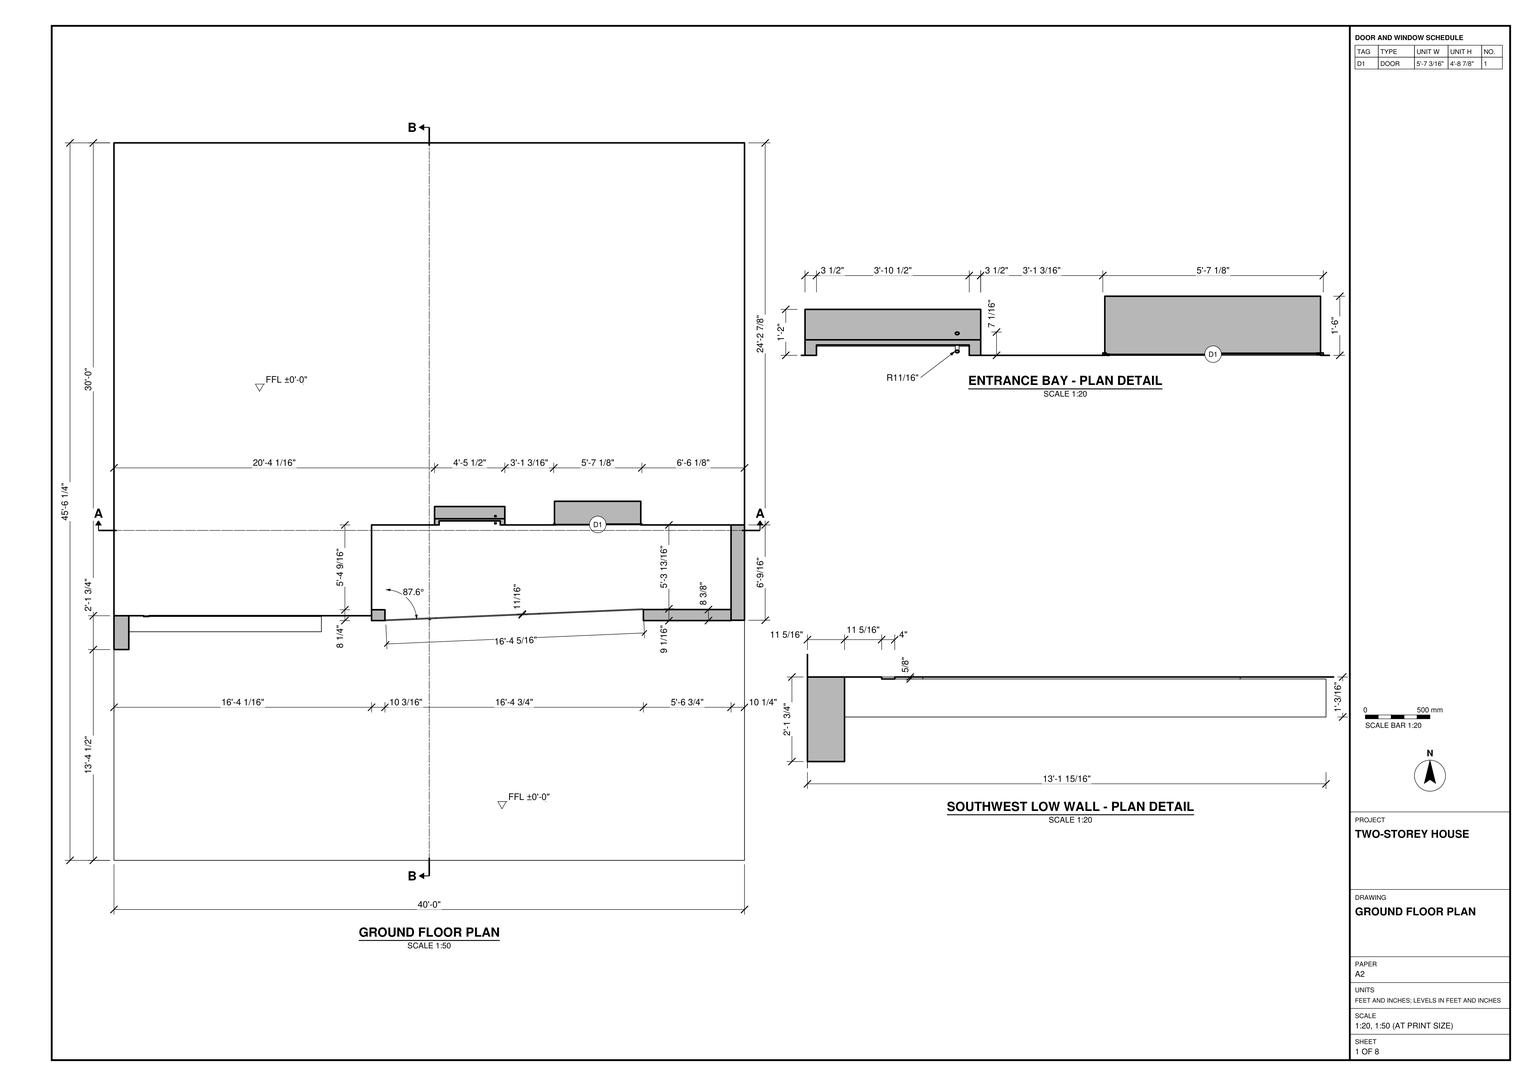
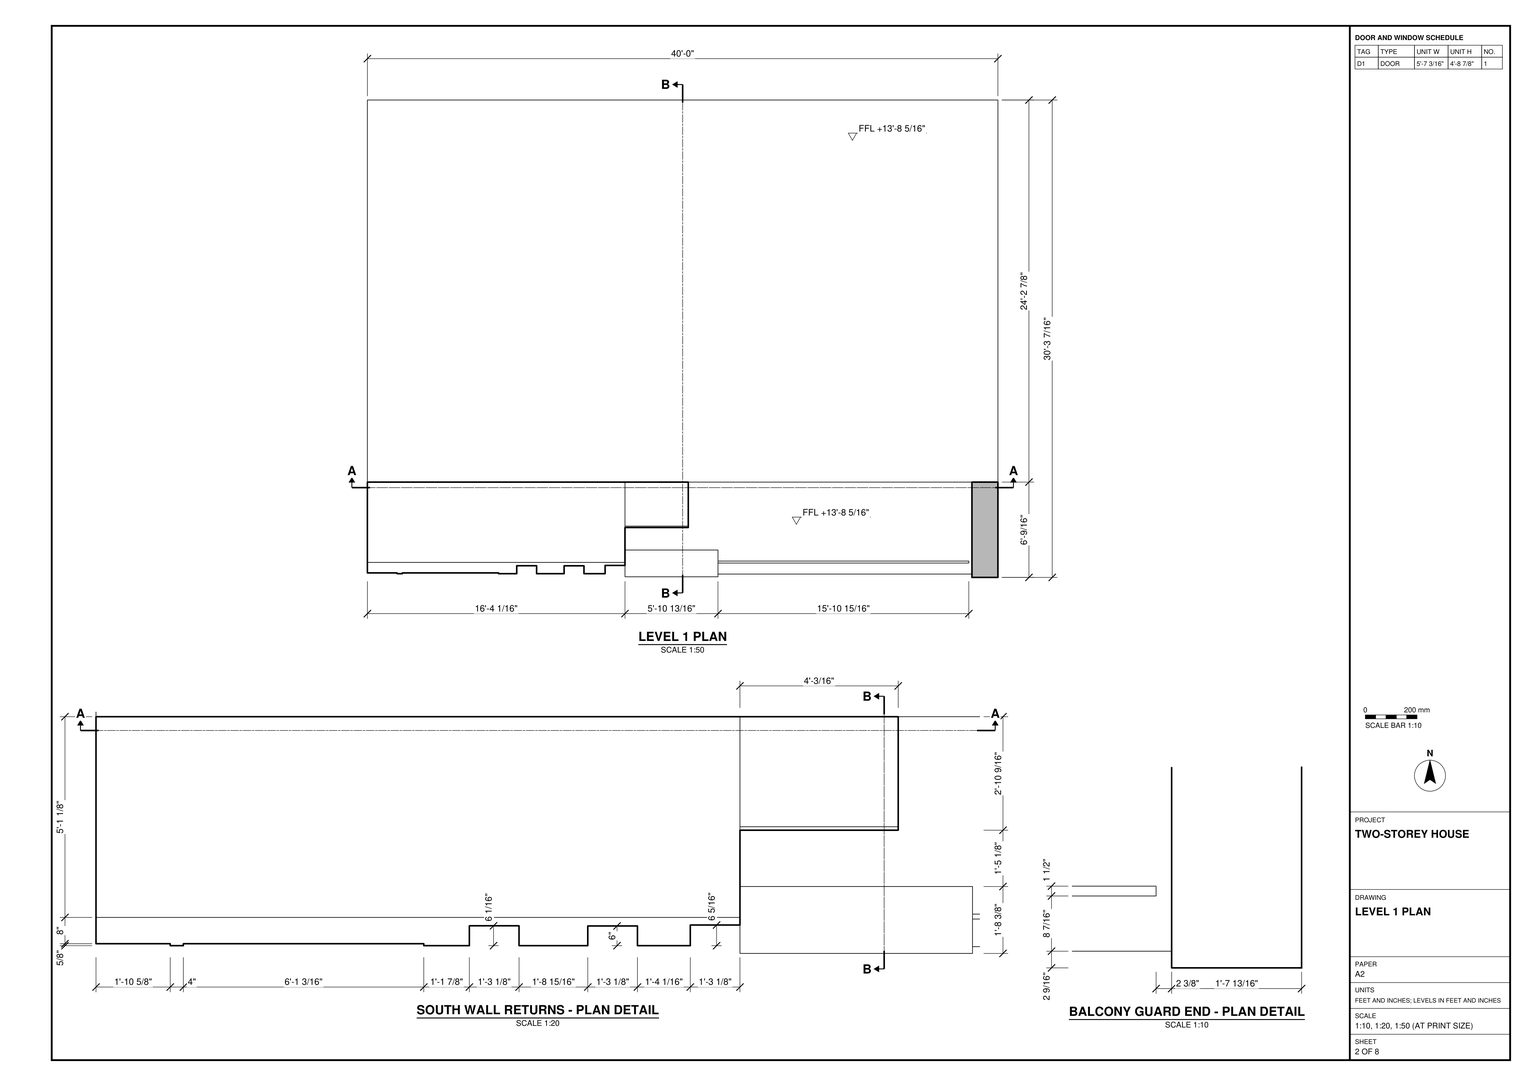
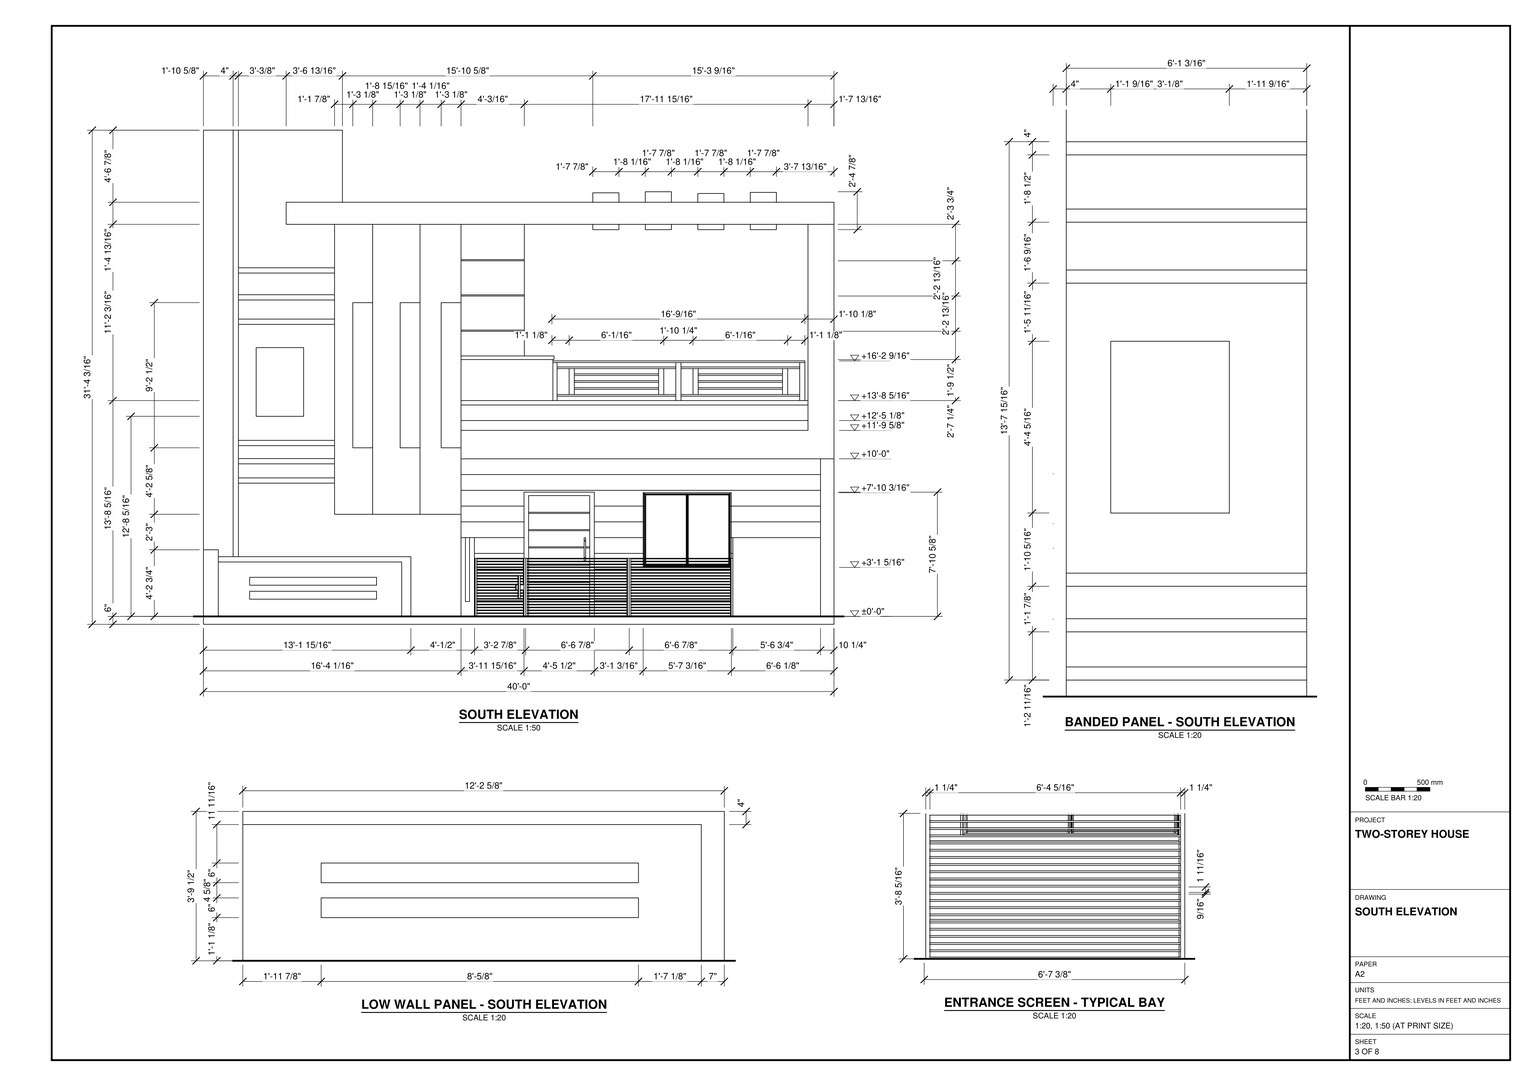
Model the two-storey house in SketchUp using task_files/diagram_01.pdf. Work in feet and inches. The overall model is 40'-0" wide, 45'-6 1/4" deep and 31'-4 3/16" high, including the base slab. Set the ground floor at ±0'-0" and the upper floor at +13'-8 5/16".

Use the plans to distinguish the full base slab from the smaller house footprint. Match the wall thicknesses, returns, floor slabs and roof outline to the drawings. On the south side, set the entrance back from the screen and follow the slight angle of the screen in plan. Include the framed sliding door, the horizontal slats and the separate low wall at the southwest corner with its two long inset strips.

Use the south elevation together with the upper-floor plan to shape the tall banded panel, the projecting vertical wall returns and the open balcony bay. Model the balcony slab and guard, the end support and the long overhead member with its short crosspieces. Include stairs, built-in joinery and main furniture only where shown. Decor and loose items may be any suitable library components.

Keep shell elements such as walls, slabs and roof separate as groups or components, and do the same for each furniture or joinery piece. Use components for repeated parts. Save one SketchUp model as output_files/two_storey_house_with_its_screened_entrance_and_balcony.skp.

# SketchUp Ruby script. Lengths in inches.
U = 1.inch
M = Sketchup.active_model
def pt(a) = Geom::Point3d.new(a.map { |v| v * U })
def face(e, loops, mat)
  f = e.add_face(loops[0].map { |a| pt(a) })
  loops[1..].each { |l| e.add_face(l.map { |a| pt(a) }).erase! }
  f.material = f.back_material = mat if mat
  f
end
# faces: each face lists its corners as indices into pts; further lists are holes
def faces(e, pts, list, mat = nil) = list.each { |f| face(e, (f[0].is_a?(Array) ? f : [f]).map { |l| l.map { |i| pts[i] } }, mat) }
# xy, xz, yz: faces in a plane at the given z, y or x. An outline is a flat list of corners, or four numbers for a rectangle; further outlines are holes
def ring(l) = l.size == 4 ? [[l[0], l[1]], [l[2], l[1]], [l[2], l[3]], [l[0], l[3]]] : l.each_slice(2).to_a
def flat(e, list, mat, &to3) = list.each { |f| face(e, (f[0].is_a?(Array) ? f : [f]).map { |l| ring(l).map { |u, v| to3.(u, v) } }, mat) }
def xy(e, z, list, mat = nil) = flat(e, list, mat) { |x, y| [x, y, z] }
def xz(e, y, list, mat = nil) = flat(e, list, mat) { |x, z| [x, y, z] }
def yz(e, x, list, mat = nil) = flat(e, list, mat) { |y, z| [x, y, z] }
def lines(e, pts, list) = list.each { |a, b| e.add_line(pt(pts[a]), pt(pts[b])) }
# prism: a flat outline (further loops are holes) pulled along v
def prism(e, loops, v, mat = nil)
  f = face(e, loops, mat); d = Geom::Vector3d.new(v.map { |x| x * U })
  f.pushpull(f.normal.samedirection?(d) ? d.length : -d.length)
end
def box(e, o, s, mat = nil) = prism(e, [[o, [o[0] + s[0], o[1], o[2]], [o[0] + s[0], o[1] + s[1], o[2]], [o[0], o[1] + s[1], o[2]]]], [0, 0, s[2]], mat)
def at(x, y, z, deg = 0) = Geom::Transformation.translation(pt([x, y, z])) * Geom::Transformation.rotation(ORIGIN, Z_AXIS, deg.degrees)
def axes(o, x, y, z) = Geom::Transformation.new([*x, 0, *y, 0, *z, 0, *pt(o).to_a, 1])
def part(name) = M.definitions.add(name)
# library, detail: a bought-in or finely detailed component or shape, given as its bounding box
def library(name, o, s) = part(name).tap { |d| box(d.entities, o, s) }
def detail(e, o, s) = box(e.add_group.entities, o, s)
def put(e, d, t, mat = nil) = e.add_instance(d, t).tap { |i| i.material = mat if mat }
def group(e, t, mat = nil) = e.add_group.tap { |g| g.transformation = t; g.material = mat if mat }.entities
root = M.entities
M.materials.add("Glass_Tinted_Gray").color = [0, 0, 0]
M.materials["Glass_Tinted_Gray"].alpha = 0.125
M.materials.add("Painted Metal Railing").color = [35, 35, 35]
M.materials.add("[0042_Sienna]").color = [160, 82, 45]
M.materials.add("[0129_WhiteSmoke]").color = [245, 245, 245]
M.materials.add("[0135_DarkGray]").color = [81, 81, 81]
M.materials.add("[Carrera Marble]").color = [207, 207, 207]
M.materials.add("[Color G01]").color = [204, 255, 204]
M.materials.add("[Color H01]").color = [204, 255, 255]
M.materials.add("[Color M00]").color = [255, 255, 255]
M.materials.add("[Color M04]").color = [142, 142, 142]
M.materials.add("[Color M05]").color = [114, 114, 114]
M.materials.add("[Color M06]").color = [86, 86, 86]
M.materials.add("[Color M07]").color = [58, 58, 58]
M.materials.add("[Metal_Corrogated_Shiny]2").color = [114, 114, 114]
M.materials.add("[Mirror 02]").color = [229, 229, 229]
M.materials.add("[Sandstone]").color = [118, 81, 52]
M.materials.add("[Terrazzo Light Blue]").color = [196, 214, 227]
M.materials.add("[Wood Veneer 01]").color = [119, 70, 35]
M.materials.add("[Wood Veneer 01]1").color = [120, 70, 37]
c1 = part("Post")
box(c1.entities,[-0.75,-0.75,0],[1.5,1.5,34.5],"Painted Metal Railing")
c2 = part("Group43\#1")
box(c2.entities,[-0.75,0,0],[1.5,73.5,1.5],"Painted Metal Railing")
c3 = part("Group46\#1")
box(c3.entities,[-0.75,0.75,0],[1.5,34.5,1.5],"Painted Metal Railing")
c4 = part("Group49\#1")
box(c4.entities,[-0.75,0.75,0],[1.5,34.5,1.5],"Painted Metal Railing")
c5 = part("Group52\#1")
box(c5.entities,[-0.75,0.75,0],[1.5,34.5,1.5],"Painted Metal Railing")
c6 = part("Group55\#1")
box(c6.entities,[-0.75,0.75,0],[1.5,34.5,1.5],"Painted Metal Railing")
c7 = part("Inner Post")
box(c7.entities,[-0.75,-0.75,0],[1.5,1.5,23.5],"Painted Metal Railing")
c8 = part("Group59\#1")
box(c8.entities,[-0.75,0.75,0],[1.5,24.5,1.5],"Painted Metal Railing")
c9 = part("Group62\#1")
box(c9.entities,[-0.75,0.75,0],[1.5,24.5,1.5],"Painted Metal Railing")
c10 = part("Group65\#1")
box(c10.entities,[-0.75,0.75,0],[1.5,24.5,1.5],"Painted Metal Railing")
c11 = part("Inner Posts and Rails\#2")
put(c11.entities,c7,at(0,0,0,90))
put(c11.entities,c7,at(0,26,0,90))
put(c11.entities,c8,at(0,0,4.75))
put(c11.entities,c9,at(0,0,11))
put(c11.entities,c10,at(0,0,17.25))
c12 = part("Group69\#1")
box(c12.entities,[-0.75,0.75,0],[1.5,24.5,1.5],"Painted Metal Railing")
c13 = part("Group72\#1")
box(c13.entities,[-0.75,0.75,0],[1.5,24.5,1.5],"Painted Metal Railing")
c14 = part("Group75\#1")
box(c14.entities,[-0.75,0.75,0],[1.5,24.5,1.5],"Painted Metal Railing")
c15 = part("Inner Posts and Rails\#3")
put(c15.entities,c7,at(0,0,0,90))
put(c15.entities,c7,at(0,26,0,90))
put(c15.entities,c12,at(0,0,4.75))
put(c15.entities,c13,at(0,0,11))
put(c15.entities,c14,at(0,0,17.25))
c16 = part("Railing Assembly 14\#1")
put(c16.entities,c1,at(0,0,0))
put(c16.entities,c1,at(36,0,0))
put(c16.entities,c1,at(72,0,0))
put(c16.entities,c2,at(-0.75,0,34.5,-90))
put(c16.entities,c3,at(0,0,4,-90))
put(c16.entities,c4,at(36,0,4,-90))
put(c16.entities,c5,at(0,0,29,-90))
put(c16.entities,c6,at(36,0,29,-90))
put(c16.entities,c11,at(5,0,5.5,-90))
put(c16.entities,c15,at(41,0,5.5,-90))
c17 = part("Group\#1")
xy(c17.entities,0,[[0.39,1.57,0.29,1.59,0.2,1.63,0.12,1.69,0.05,1.77,0.01,1.87,0,1.97,0.01,2.07,0.05,2.17,0.12,2.25,0.2,2.31,0.29,2.35,0.39,2.36,0.5,2.35,0.59,2.31,0.67,2.25,0.73,2.17,0.77,2.07,0.79,1.97,0.77,1.87,0.73,1.77,0.67,1.69,0.59,1.63,0.5,1.59],[0.39,13.39,0.29,13.4,0.2,13.4375,0.12,13.5,0.05,13.58,0.01,13.68,0,13.78,0.01,13.88,0.05,13.98,0.12,14.06,0.2,14.12,0.29,14.16,0.39,14.17,0.5,14.16,0.59,14.12,0.67,14.06,0.73,13.98,0.77,13.88,0.79,13.78,0.77,13.68,0.73,13.58,0.67,13.5,0.59,13.4375,0.5,13.4]])
xy(c17.entities,1.97,[[0.39,1.57,0.39,2.36,0.29,2.35,0.2,2.31,0.12,2.25,0.05,2.17,0.01,2.07,0,1.97,0.01,1.87,0.05,1.77,0.12,1.69,0.2,1.63,0.29,1.59],[0.39,1.57,0.5,1.59,0.59,1.63,0.67,1.69,0.73,1.77,0.77,1.87,0.79,1.97,0.77,2.07,0.73,2.17,0.67,2.25,0.59,2.31,0.5,2.35,0.39,2.36],[0.39,13.39,0.39,14.17,0.29,14.16,0.2,14.12,0.12,14.06,0.05,13.98,0.01,13.88,0,13.78,0.01,13.68,0.05,13.58,0.12,13.5,0.2,13.4375,0.29,13.4],[0.39,13.39,0.5,13.4,0.59,13.4375,0.67,13.5,0.73,13.58,0.77,13.68,0.79,13.78,0.77,13.88,0.73,13.98,0.67,14.06,0.59,14.12,0.5,14.16,0.39,14.17]])
xz(c17.entities,0,[[0.39,1.57,0.5,1.59,0.59,1.63,0.67,1.69,0.73,1.77,0.77,1.87,0.79,1.97,0.77,2.07,0.73,2.17,0.67,2.25,0.59,2.31,0.5,2.35,0.39,2.36,0.29,2.35,0.2,2.31,0.12,2.25,0.05,2.17,0.01,2.07,0,1.97,0.01,1.87,0.05,1.77,0.12,1.69,0.2,1.63,0.29,1.59]])
xz(c17.entities,15.75,[[0.39,1.57,0.29,1.59,0.2,1.63,0.12,1.69,0.05,1.77,0.01,1.87,0,1.97,0.01,2.07,0.05,2.17,0.12,2.25,0.2,2.31,0.29,2.35,0.39,2.36,0.5,2.35,0.59,2.31,0.67,2.25,0.73,2.17,0.77,2.07,0.79,1.97,0.77,1.87,0.73,1.77,0.67,1.69,0.59,1.63,0.5,1.59]])
p = [[0.12,1.69,0],[0.2,1.63,0],[0.2,1.63,1.63],[0.2,1.63,1.97],[0.12,1.69,1.97],[0.12,1.69,1.69],
  [0.29,1.59,0],[0.29,1.59,1.59],[0.29,1.59,1.97],[0.39,1.57,0],[0.39,1.57,1.57],[0.39,1.57,1.97],
  [0.5,1.59,0],[0.5,1.59,1.59],[0.5,1.59,1.97],[0.59,1.63,0],[0.59,1.63,1.63],[0.59,1.63,1.97],
  [0.67,1.69,0],[0.67,1.69,1.69],[0.67,1.69,1.97],[0.05,1.77,0],[0.05,1.77,1.97],[0.05,1.77,1.77],
  [0.73,1.77,0],[0.73,1.77,1.77],[0.73,1.77,1.97],[0.01,1.87,0],[0.01,1.87,1.97],[0.01,1.87,1.87],
  [0.77,1.87,0],[0.77,1.87,1.87],[0.77,1.87,1.97],[0,1.97,0],[0,1.97,1.97],[0.79,1.97,0],
  [0.79,1.97,1.97],[0.01,2.07,0],[0.01,2.07,1.97],[0.01,2.07,1.87],[0.77,2.07,0],[0.77,2.07,1.87],
  [0.77,2.07,1.97],[0.05,2.17,0],[0.05,2.17,1.97],[0.05,2.17,1.77],[0.73,2.17,0],[0.73,2.17,1.77],
  [0.73,2.17,1.97],[0.12,2.25,0],[0.12,2.25,1.97],[0.12,2.25,1.69],[0.2,2.31,0],[0.2,2.31,1.97],
  [0.2,2.31,1.63],[0.67,2.25,0],[0.59,2.31,0],[0.59,2.31,1.63],[0.59,2.31,1.97],[0.67,2.25,1.97],
  [0.67,2.25,1.69],[0.29,2.35,0],[0.29,2.35,1.97],[0.29,2.35,1.59],[0.39,2.36,0],[0.39,2.36,1.97],
  [0.39,2.36,1.57],[0.5,2.35,0],[0.5,2.35,1.97],[0.5,2.35,1.59],[0.12,13.5,0],[0.2,13.4375,0],
  [0.2,13.4375,1.63],[0.2,13.4375,1.97],[0.12,13.5,1.97],[0.12,13.5,1.69],[0.29,13.4,0],[0.29,13.4,1.59],
  [0.29,13.4,1.97],[0.39,13.39,0],[0.39,13.39,1.57],[0.39,13.39,1.97],[0.5,13.4,0],[0.5,13.4,1.59],
  [0.5,13.4,1.97],[0.59,13.4375,0],[0.59,13.4375,1.63],[0.59,13.4375,1.97],[0.67,13.5,0],[0.67,13.5,1.69],
  [0.67,13.5,1.97],[0.05,13.58,0],[0.05,13.58,1.97],[0.05,13.58,1.77],[0.73,13.58,0],[0.73,13.58,1.77],
  [0.73,13.58,1.97],[0.01,13.68,0],[0.01,13.68,1.97],[0.01,13.68,1.87],[0.77,13.68,0],[0.77,13.68,1.87],
  [0.77,13.68,1.97],[0,13.78,0],[0,13.78,1.97],[0.79,13.78,0],[0.79,13.78,1.97],[0.01,13.88,0],
  [0.01,13.88,1.97],[0.01,13.88,1.87],[0.77,13.88,0],[0.77,13.88,1.87],[0.77,13.88,1.97],[0.05,13.98,0],
  [0.05,13.98,1.97],[0.05,13.98,1.77],[0.73,13.98,0],[0.73,13.98,1.77],[0.73,13.98,1.97],[0.12,14.06,0],
  [0.12,14.06,1.97],[0.12,14.06,1.69],[0.67,14.06,0],[0.67,14.06,1.69],[0.67,14.06,1.97],[0.2,14.12,0],
  [0.2,14.12,1.97],[0.2,14.12,1.63],[0.29,14.16,0],[0.29,14.16,1.97],[0.29,14.16,1.59],[0.59,14.12,0],
  [0.5,14.16,0],[0.5,14.16,1.59],[0.5,14.16,1.97],[0.59,14.12,1.97],[0.59,14.12,1.63],[0.39,14.17,0],
  [0.39,14.17,1.97],[0.39,14.17,1.57],[0.12,15.75,1.69],[0.2,15.75,1.63],[0.2,0,1.63],[0.12,0,1.69],
  [0.29,15.75,1.59],[0.29,0,1.59],[0.39,15.75,1.57],[0.39,13.78,1.57],[0.39,1.97,1.57],[0.39,0,1.57],
  [0.5,15.75,1.59],[0.5,0,1.59],[0.59,15.75,1.63],[0.59,0,1.63],[0.67,15.75,1.69],[0.67,0,1.69],
  [0.05,15.75,1.77],[0.05,0,1.77],[0.73,15.75,1.77],[0.73,0,1.77],[0.01,15.75,1.87],[0.01,0,1.87],
  [0.77,15.75,1.87],[0.77,0,1.87],[0,15.75,1.97],[0,0,1.97],[0.79,15.75,1.97],[0.79,0,1.97],
  [0.01,15.75,2.07],[0.01,0,2.07],[0.77,15.75,2.07],[0.77,0,2.07],[0.05,15.75,2.17],[0.05,0,2.17],
  [0.73,15.75,2.17],[0.73,0,2.17],[0.12,15.75,2.25],[0.12,0,2.25],[0.2,15.75,2.31],[0.2,0,2.31],
  [0.67,15.75,2.25],[0.59,15.75,2.31],[0.59,0,2.31],[0.67,0,2.25],[0.29,15.75,2.35],[0.29,0,2.35],
  [0.39,15.75,2.36],[0.39,0,2.36],[0.5,15.75,2.35],[0.5,0,2.35],[0.39,1.97,1.97],[0.39,13.78,0],
  [0.39,1.97,0],[0.39,13.78,1.97],[0.39,0,1.97],[0.39,15.75,1.97]]
faces(c17.entities,p,[[0,1,2,3,4,5],[1,6,7,8,3,2],[6,9,10,11,8,7],[9,12,13,14,11,10],[12,15,16,17,14,13],[15,18,19,20,17,16],[21,0,5,4,22,23],[18,24,25,26,20,19],
  [27,21,23,22,28,29],[24,30,31,32,26,25],[33,27,29,28,34],[30,35,36,32,31],[37,33,34,38,39],[35,40,41,42,36],[43,37,39,38,44,45],[40,46,47,48,42,41],
  [49,43,45,44,50,51],[52,49,51,50,53,54],[55,56,57,58,59,60],[46,55,60,59,48,47],[61,52,54,53,62,63],[64,61,63,62,65,66],[67,64,66,65,68,69],[56,67,69,68,58,57],
  [70,71,72,73,74,75],[71,76,77,78,73,72],[76,79,80,81,78,77],[79,82,83,84,81,80],[82,85,86,87,84,83],[85,88,89,90,87,86],[91,70,75,74,92,93],[88,94,95,96,90,89],
  [97,91,93,92,98,99],[94,100,101,102,96,95],[103,97,99,98,104],[100,105,106,102,101],[107,103,104,108,109],[105,110,111,112,106],[113,107,109,108,114,115],[110,116,117,118,112,111],
  [119,113,115,114,120,121],[116,122,123,124,118,117],[125,119,121,120,126,127],[128,125,127,126,129,130],[131,132,133,134,135,136],[122,131,136,135,124,123],[137,128,130,129,138,139],[132,137,139,138,134,133],
  [140,141,127,72,54,2,142,143,5,51,75,121],[141,144,130,77,63,7,145,142,2,54,72,127],[144,146,139,147,80,66,148,10,149,145,7,63,77,130],[146,150,133,83,69,13,151,149,10,148,66,80,147,139],[150,152,136,86,57,16,153,151,13,69,83,133],[152,154,123,89,60,19,155,153,16,57,86,136],[156,140,121,75,51,5,143,157,23,45,93,115],[154,158,117,95,47,25,159,155,19,60,89,123],
  [160,156,115,93,45,23,157,161,29,39,99,109],[158,162,111,101,41,31,163,159,25,47,95,117],[164,160,109,99,39,29,161,165,34,104],[162,166,106,36,167,163,31,41,101,111],[168,164,104,34,165,169],[166,170,171,167,36,106],[172,168,169,173],[170,174,175,171],
  [176,172,173,177],[178,176,177,179],[180,181,182,183],[174,180,183,175],[184,178,179,185],[186,184,185,187],[188,186,187,189],[181,188,189,182]])
lines(c17.entities,p,[[190,148],[191,147],[148,192],[147,193],[11,194],[138,195],[81,65]])
c18 = part("3+80")
p = [[0,0,0],[1,0,0],[1,1,0]]
lines(c18.entities,p,[[0,1],[1,2],[2,0]])
g1 = group(c18.entities,at(0,0.01,-0.01))
g2 = group(g1,at(0,0,0))
xy(g2,0.01,[[0,-4.72,2.36,0],[33.86,-4.72,36.22,0],[2.36,-1.57,33.86,0]])
xy(g2,11.42,[[2.36,-1.97,33.86,-1.57]],"[Color M04]")
xy(g2,12.2,[[2.36,-1.97,33.86,-1.57]],"[Color M04]")
xy(g2,23.23,[[2.36,-1.97,33.86,-1.57]],"[Color M04]")
xy(g2,24.02,[[2.36,-1.97,33.86,-1.57]],"[Color M04]")
xy(g2,35.04,[[2.36,-1.97,33.86,-1.57]],"[Color M04]")
xy(g2,35.83,[[2.36,-1.97,33.86,-1.57]],"[Color M04]")
xy(g2,46.85,[[2.36,-2.36,33.86,-1.57]],"[Color M04]")
xy(g2,47.64,[[2.36,-2.36,33.86,-1.57]],"[Color M04]")
xy(g2,58.66,[[2.36,-2.36,33.86,-1.57]],"[Color M04]")
xy(g2,59.45,[[2.36,-2.36,33.86,-1.57]],"[Color M04]")
xy(g2,70.47,[[2.36,-2.36,33.86,-1.57]],"[Color M04]")
xy(g2,71.26,[[2.36,-2.36,33.86,-1.57]],"[Color M04]")
xy(g2,82.68,[[2.36,-4.72,33.86,-1.57]],"[Wood Veneer 01]")
xy(g2,85.04,[[0,-4.72,36.22,0]],"[Wood Veneer 01]")
xz(g2,-4.72,[[0,0.01,0,85.04,36.22,85.04,36.22,0.01,33.86,0.01,33.86,82.68,2.36,82.68,2.36,0.01]],"[Wood Veneer 01]")
xz(g2,-2.36,[[2.36,46.85,33.86,47.64],[2.36,58.66,33.86,59.45],[2.36,70.47,33.86,71.26]],"[Color M04]")
xz(g2,-1.97,[[2.36,11.42,33.86,12.2],[2.36,23.23,33.86,24.02],[2.36,35.04,33.86,35.83]],"[Color M04]")
xz(g2,-1.57,[[2.36,0.01,33.86,11.42],[2.36,12.2,33.86,23.23],[2.36,24.02,33.86,35.04],[2.36,35.83,33.86,46.85],[2.36,47.64,33.86,58.66],
  [2.36,59.45,33.86,70.47],[2.36,71.26,33.86,82.68]],"[Wood Veneer 01]")
xz(g2,0,[[0,0.01,2.36,0.01,2.36,82.68,33.86,82.68,33.86,0.01,36.22,0.01,36.22,85.04,0,85.04],[2.36,0.01,33.86,82.68]],"[Wood Veneer 01]")
yz(g2,0,[[-4.72,0.01,0,85.04]],"[Wood Veneer 01]")
yz(g2,2.36,[[-4.72,0.01,-4.72,82.68,-1.57,82.68,-1.57,71.26,-2.36,71.26,-2.36,70.47,-1.57,70.47,-1.57,59.45,-2.36,59.45,-2.36,58.66,-1.57,58.66,-1.57,47.64,-2.36,47.64,-2.36,46.85,-1.57,46.85,-1.57,35.83,-1.97,35.83,-1.97,35.04,-1.57,35.04,-1.57,24.02,-1.97,24.02,-1.97,23.23,-1.57,23.23,-1.57,12.2,-1.97,12.2,-1.97,11.42,-1.57,11.42,-1.57,0.01]],"[Wood Veneer 01]")
yz(g2,33.86,[[-4.72,0.01,-1.57,0.01,-1.57,11.42,-1.97,11.42,-1.97,12.2,-1.57,12.2,-1.57,23.23,-1.97,23.23,-1.97,24.02,-1.57,24.02,-1.57,35.04,-1.97,35.04,-1.97,35.83,-1.57,35.83,-1.57,46.85,-2.36,46.85,-2.36,47.64,-1.57,47.64,-1.57,58.66,-2.36,58.66,-2.36,59.45,-1.57,59.45,-1.57,70.47,-2.36,70.47,-2.36,71.26,-1.57,71.26,-1.57,82.68,-4.72,82.68]],"[Wood Veneer 01]")
yz(g2,36.22,[[-4.72,0.01,0,85.04]],"[Wood Veneer 01]")
p = [[0,0,0],[0,0,0.01]]
lines(g2,p,[[0,1]])
put(g1,c17,axes([30.98,0,38.01],[1,0,0],[0,0,1],[0,1,0]),"[Color M04]")
put(g1,c17,axes([30.98,-1.57,38.01],[1,0,0],[0,0,1],[0,-1,0]),"[Color M04]")
c19 = part("PENTEK_RP Fineline 50S_Sliding_DoorCase_E1")
box(c19.entities,[0,0,0],[1.51,3.66,99.27],"[0135_DarkGray]")
c20 = part("PENTEK_RP Fineline 50S_SlidingDooe_Case_E2")
box(c20.entities,[0,0,0],[96.25,3.66,1.51],"[0135_DarkGray]")
c21 = part("pentek_RP Fineline 50S_SlidingDoor_Case")
put(c21.entities,c19,at(97.76,0,0))
put(c21.entities,c20,at(1.51,0,0))
put(c21.entities,c19,at(0,0,0))
put(c21.entities,c20,at(1.51,0,97.76))
c22 = part("PENTEK_RP Fineline 50S_SlidingDoor_GlazingBead_2")
box(c22.entities,[0,0,0],[0.56,0.59,94.39],"[0135_DarkGray]")
c23 = part("PENTEK_RP Fineline 50S_SlidingDoor_Glass")
box(c23.entities,[0,0,0],[46.58,0.16,94.39],"Glass_Tinted_Gray")
c24 = part("PENTEK_RP Fineline 50S_SlidingDoor_GlazingBead")
box(c24.entities,[0,0,0],[45.47,0.59,0.56],"[0135_DarkGray]")
c25 = part("PENTEK_RP Fineline 50S_SlidingDoor_Leaf_E1")
xy(c25.entities,0,[[0,0,0.93,1.97],[0.93,1.57,1.49,1.97]],"[0135_DarkGray]")
xy(c25.entities,96.25,[[0,0,0.93,0,0.93,1.57,1.49,1.57,1.49,1.97,0,1.97]],"[0135_DarkGray]")
xz(c25.entities,0,[[0,0,0.93,96.25]],"[0135_DarkGray]")
xz(c25.entities,1.57,[[0.93,0,1.49,95.32],[0.93,95.32,1.49,96.25]],"[0135_DarkGray]")
xz(c25.entities,1.97,[[0,0,1.49,96.25]],"[0135_DarkGray]")
yz(c25.entities,0,[[0,0,1.97,96.25]],"[0135_DarkGray]")
yz(c25.entities,0.93,[[0,0,1.57,0.93],[0,0.93,1.57,95.32],[0,95.32,1.57,96.25]],"[0135_DarkGray]")
yz(c25.entities,1.49,[[1.57,0,1.97,95.32],[1.57,95.32,1.97,96.25]],"[0135_DarkGray]")
c26 = part("PENTEK_RP Fineline 50S_SlidingDoor_Leaf_E2")
xy(c26.entities,0,[[0,0,0,1.57,0.56,1.57,0.56,1.97,46.02,1.97,46.02,1.57,46.58,1.57,46.58,0]],"[0135_DarkGray]")
xy(c26.entities,0.93,[[0,0,46.58,1.57]],"[0135_DarkGray]")
xy(c26.entities,1.49,[[0.56,1.57,46.02,1.97]],"[0135_DarkGray]")
xz(c26.entities,0,[[0,0,46.58,0.93]],"[0135_DarkGray]")
xz(c26.entities,1.57,[[0,0,0.56,0.93],[46.02,0,46.58,0.93],[0.56,0.93,46.02,1.49]],"[0135_DarkGray]")
xz(c26.entities,1.97,[[0.56,0,46.02,1.49]],"[0135_DarkGray]")
yz(c26.entities,0,[[0,0,1.57,0.93]],"[0135_DarkGray]")
yz(c26.entities,0.56,[[1.57,0,1.97,0.93],[1.57,0.93,1.97,1.49]],"[0135_DarkGray]")
yz(c26.entities,46.02,[[1.57,0,1.97,0.93],[1.57,0.93,1.97,1.49]],"[0135_DarkGray]")
yz(c26.entities,46.58,[[0,0,1.57,0.93]],"[0135_DarkGray]")
c27 = part("PENTEK_RP Fineline S_SlidingDoor_Leaf1")
put(c27.entities,c22,at(0.93,0,0.93))
put(c27.entities,c22,at(46.96,0,0.93))
put(c27.entities,c23,at(1.49,1.42,0.93))
put(c27.entities,c24,at(1.49,0,0.93))
put(c27.entities,c23,at(1.49,0.59,0.93),"[Terrazzo Light Blue]")
put(c27.entities,c25,at(0,0,0))
put(c27.entities,c25,axes([48.44,0,0],[-1,0,0],[0,1,0],[0,0,1]))
put(c27.entities,c26,axes([0.93,0,96.25],[1,0,0],[0,1,0],[0,0,-1]))
put(c27.entities,c26,at(0.93,0,0))
put(c27.entities,c24,at(1.49,0,94.77))
c28 = part("PENTEK_RP Fineline 50S_SlidingDoor_Leaf2")
put(c28.entities,c23,at(1.49,1.42,0.93))
put(c28.entities,c24,at(1.49,0,94.77))
put(c28.entities,c22,at(46.96,0,0.93))
put(c28.entities,c23,at(1.49,0.59,0.93),"[Mirror 02]")
put(c28.entities,c22,at(0.93,0,0.93))
put(c28.entities,c25,at(0,0,0))
put(c28.entities,c25,axes([48.44,0,0],[-1,0,0],[0,1,0],[0,0,1]))
put(c28.entities,c24,at(1.49,0,0.93))
put(c28.entities,c26,axes([0.93,0,96.25],[1,0,0],[0,1,0],[0,0,-1]))
put(c28.entities,c26,at(0.93,0,0))
c29 = part("PENTEK - Slimmest Steel Sliding Door / Window\#1")
put(c29.entities,c21,at(0,-1.88,-0.09))
put(c29.entities,c27,at(1.51,-2.27,1.42))
put(c29.entities,c28,at(49.32,-0.3,1.42))
c30 = part("Screen slat")
box(c30.entities,[0,0,0],[70.44,1.18,1.18])
c31 = part("Screen upright")
box(c31.entities,[0,0,0],[1.18,1.18,38.9])
c32 = part("Componente\#10")
box(c32.entities,[0,0,0],[5.39,1.18,8.54])
c33 = part("Screen panel frame")
prism(c33.entities,[[[0,0,0],[72.8,0,0],[72.8,0,98.43],[0,0,98.43]],[[1.18,0,97.24],[71.62,0,97.24],[71.62,0,1.18],[1.18,0,1.18]]],[0,1.18,0])
c34 = part("Slatted screen panel")
put(c34.entities,c30,at(1.18,0,92.38))
put(c34.entities,c30,at(1.18,0,53.48))
put(c34.entities,c30,at(1.18,0,48.62))
put(c34.entities,c30,at(1.18,0,43.76))
put(c34.entities,c30,at(1.18,0,38.9))
put(c34.entities,c30,at(1.18,0,34.04))
put(c34.entities,c30,at(1.18,0,29.17))
put(c34.entities,c30,at(1.18,0,24.3125))
put(c34.entities,c30,at(1.18,0,4.86))
put(c34.entities,c33,at(0,0,0))
put(c34.entities,c30,at(1.18,0,82.66))
put(c34.entities,c30,at(1.18,0,87.52))
put(c34.entities,c30,at(1.18,0,68.07))
put(c34.entities,c30,at(1.18,0,19.45))
put(c34.entities,c30,at(1.18,0,72.93))
put(c34.entities,c30,at(1.18,0,14.59))
put(c34.entities,c30,at(1.18,0,63.21))
put(c34.entities,c30,at(1.18,0,9.72))
put(c34.entities,c30,at(1.18,0,58.35))
put(c34.entities,c30,at(1.18,0,77.8))
c35 = part("Entrance gate frame")
prism(c35.entities,[[[0,0,0],[35.43,0,0],[35.43,0,98.43],[0,0,98.43]],[[1.18,0,1.18],[1.18,0,97.24],[34.25,0,97.24],[34.25,0,1.18]]],[0,1.18,0])
c36 = part("Screen slat \#1")
box(c36.entities,[0,0,0],[70.44,1.18,1.18])
c37 = part("Slatted entrance screen")
put(c37.entities,c30,axes([0.56,1.57,92.38],[0.4241,0.20138,0],[-0.42894,0.90334,0],[0,0,1]),"[Metal_Corrogated_Shiny]2")
put(c37.entities,c30,axes([0.56,1.57,53.48],[0.4241,0.20138,0],[-0.42894,0.90334,0],[0,0,1]),"[Metal_Corrogated_Shiny]2")
put(c37.entities,c30,axes([0.56,1.57,4.86],[0.4241,0.20138,0],[-0.42894,0.90334,0],[0,0,1]),"[Metal_Corrogated_Shiny]2")
put(c37.entities,c31,at(27.14,12.89,30.35,25.4),"[Metal_Corrogated_Shiny]2")
put(c37.entities,c30,axes([0.56,1.57,24.3125],[0.4241,0.20138,0],[-0.42894,0.90334,0],[0,0,1]),"[Metal_Corrogated_Shiny]2")
put(c37.entities,c32,at(25.56,13.45,44.94,25.4),"[Metal_Corrogated_Shiny]2")
put(c37.entities,c30,axes([0.56,1.57,82.66],[0.4241,0.20138,0],[-0.42894,0.90334,0],[0,0,1]),"[Metal_Corrogated_Shiny]2")
put(c37.entities,c30,axes([0.56,1.57,63.21],[0.4241,0.20138,0],[-0.42894,0.90334,0],[0,0,1]),"[Metal_Corrogated_Shiny]2")
put(c37.entities,c30,axes([0.56,1.57,38.9],[0.4241,0.20138,0],[-0.42894,0.90334,0],[0,0,1]),"[Metal_Corrogated_Shiny]2")
put(c37.entities,c30,axes([0.56,1.57,68.07],[0.4241,0.20138,0],[-0.42894,0.90334,0],[0,0,1]),"[Metal_Corrogated_Shiny]2")
put(c37.entities,c30,axes([0.56,1.57,34.04],[0.4241,0.20138,0],[-0.42894,0.90334,0],[0,0,1]),"[Metal_Corrogated_Shiny]2")
put(c37.entities,c30,axes([0.56,1.57,77.8],[0.4241,0.20138,0],[-0.42894,0.90334,0],[0,0,1]),"[Metal_Corrogated_Shiny]2")
put(c37.entities,c30,axes([0.56,1.57,9.72],[0.4241,0.20138,0],[-0.42894,0.90334,0],[0,0,1]),"[Metal_Corrogated_Shiny]2")
put(c37.entities,c30,axes([0.56,1.57,72.93],[0.4241,0.20138,0],[-0.42894,0.90334,0],[0,0,1]),"[Metal_Corrogated_Shiny]2")
put(c37.entities,c34,at(31.5,16.27,0,25.4),"[Metal_Corrogated_Shiny]2")
put(c37.entities,c34,at(97.27,47.49,0,25.4),"[Metal_Corrogated_Shiny]2")
put(c37.entities,c30,axes([0.56,1.57,58.35],[0.4241,0.20138,0],[-0.42894,0.90334,0],[0,0,1]),"[Metal_Corrogated_Shiny]2")
put(c37.entities,c30,axes([0.56,1.57,87.52],[0.4241,0.20138,0],[-0.42894,0.90334,0],[0,0,1]),"[Metal_Corrogated_Shiny]2")
put(c37.entities,c35,at(-0.51,1.07,0,25.4),"[Metal_Corrogated_Shiny]2")
put(c37.entities,c30,axes([0.56,1.57,14.59],[0.4241,0.20138,0],[-0.42894,0.90334,0],[0,0,1]),"[Metal_Corrogated_Shiny]2")
put(c37.entities,c30,axes([0.56,1.57,19.45],[0.4241,0.20138,0],[-0.42894,0.90334,0],[0,0,1]),"[Metal_Corrogated_Shiny]2")
put(c37.entities,c30,axes([0.56,1.57,29.17],[0.4241,0.20138,0],[-0.42894,0.90334,0],[0,0,1]),"[Metal_Corrogated_Shiny]2")
put(c37.entities,c36,axes([0.56,1.57,48.62],[0.35497,0.16855,0],[-0.42894,0.90334,0],[0,0,1]),"[Metal_Corrogated_Shiny]2")
put(c37.entities,c30,axes([0.56,1.57,43.76],[0.4241,0.20138,0],[-0.42894,0.90334,0],[0,0,1]),"[Metal_Corrogated_Shiny]2")
xy(root,-6,[[0,0,480,546.25]])
xy(root,-0.34,[[150.92,174.0625,157.91,185.65]],"[Color M06]")
xy(root,0,[[0,0,480,0,480,182.8125,469.75,182.8125,469.75,182.5625,403.02,182.5625,403.02,190.96,469.75,190.96,469.75,255.375,297.54,255.375,297.54,269.375,244.04,269.375,244.04,255.375,196.09,255.375,196.09,190.79,206.28,190.79,206.28,182.5625,196.09,182.5625,196.09,186.25,11.3,186.25,11.3,160.5,0,160.5],[196.09,182.5625,206.28,186.25],[0,186.25,196.09,186.25,196.09,255.375,244.04,255.375,244.04,269.375,297.54,269.375,297.54,255.375,480,255.375,480,546.25,0,546.25],[196.09,186.25,206.28,190.79]])
xy(root,0,[[0,160.5,11.3,186.25]],"[Color M06]")
xy(root,13.14,[[35.15,185.125,131.78,186.25]],"[Color M06]")
xy(root,19.14,[[35.15,185.125,131.78,186.25]],"[Color M06]")
xy(root,23.77,[[35.15,185.125,131.78,186.25]],"[Color M06]")
xy(root,29.77,[[35.15,185.125,131.78,186.25]],"[Color M06]")
xy(root,37.68,[[335.34,255.375,401.02,273.375]])
xy(root,41.48,[[11.3,174.0625,11.3,186.25,22.6,186.25,22.6,185.65,150.92,185.65,150.92,174.0625],[22.6,185.65,26.6,186.25]],"[Color M06]")
xy(root,45.48,[[11.3,174.0625,157.91,174.0625,157.91,185.65,22.6,185.65,22.6,186.25,11.3,186.25]],"[Color M06]")
xy(root,50.74,[[0,160.5,11.3,186.25]],"[Color M00]")
xy(root,60,[[196.09,182.5625,206.28,190.79],[403.02,182.5625,469.75,190.96],[469.75,191.3125,480,255.375]])
xy(root,77.74,[[99.8125,185.65,196.09,186.25]])
xy(root,94.18,[[335.34,255.375,401.02,273.375]])
xy(root,94.625,[[244.04,255.375,297.54,269.375]])
xy(root,101.48,[[26.6,185.65,99.8125,186.25]],"[Color M06]")
xy(root,105.48,[[26.6,185.65,99.8125,186.25]],"[Color M06]")
xy(root,116.17,[[26.6,185.65,99.8125,186.25]],"[Color M06]")
xy(root,120,[[196.09,182.8125,196.09,255.375,480,255.375,480,191.3125,469.75,191.3125,469.75,182.8125],[469.75,182.8125,480,191.3125],[0,194.25,0,546.25,480,546.25,480,255.375,196.09,255.375,196.09,194.25]])
xy(root,120.17,[[26.6,185.65,99.8125,186.25]])
xy(root,128.38,[[113.6875,185.65,128.8125,191.71],[149.75,185.65,164.875,191.65],[180.96,185.65,196.09,191.9375]],"[Sandstone]")
xy(root,130.04,[[26.6,185.65,99.8125,186.25]],"[Color M06]")
xy(root,134.04,[[26.6,185.65,99.8125,186.25]])
xy(root,141.625,[[0,194.25,0,546.25,480,546.25,480,255.375,196.09,255.375,196.09,194.25]])
xy(root,141.625,[[196.09,182.8125,460.22,186.25]],"[0129_WhiteSmoke]")
xy(root,149.125,[[0,194.25,0,546.25,480,546.25,480,255.375,196.09,255.375,196.09,194.25]])
xy(root,160.9375,[[196.09,185.35,460.22,186.25]])
xy(root,164.3125,[[0,194.25,196.09,255.375],[196.09,220.8125,244.28,255.375]])
xy(root,164.3125,[[266.03,185.35,460.22,185.35,460.22,255.375,244.28,255.375,244.28,220.8125,196.09,220.8125,196.09,203.66,266.03,203.66],[0,255.375,480,546.25]],"[0129_WhiteSmoke]")
xy(root,190.25,[[196.09,220.8125,244.28,221.875]],"[Color M06]")
xy(root,191.15,[[196.09,220.8125,244.28,221.875]],"[Color M06]")
xy(root,195.5625,[[196.09,185.35,266.03,203.66]])
xy(root,195.5625,[[196.09,183.29,266.9,185.35],[266.03,185.35,266.9,203.66]],"[Color M06]")
xy(root,198.3125,[[196.09,183.29,266.9,203.66]],"[Color M06]")
xy(root,217.09,[[196.09,220.8125,244.28,222.3125]],"[Color M06]")
xy(root,217.99,[[196.09,220.8125,244.28,222.3125]],"[Color M06]")
xy(root,222.35,[[26.6,185.65,99.8125,186.25]])
xy(root,226.35,[[26.6,185.65,99.8125,186.25]],"[Color M06]")
xy(root,238.88,[[113.6875,185.65,128.8125,191.71],[149.75,185.65,164.875,191.65],[180.96,185.65,196.09,191.9375]],"[Sandstone]")
xy(root,240.92,[[26.6,185.65,99.8125,186.25]])
xy(root,243.92,[[196.09,220.8125,244.28,221.8125]],"[Color M06]")
xy(root,244.82,[[196.09,220.8125,244.28,221.8125]],"[Color M06]")
xy(root,244.92,[[26.6,185.65,99.8125,186.25]],"[Color M06]")
xy(root,261.42,[[26.6,185.65,99.8125,186.25]])
xy(root,265.42,[[26.6,185.65,99.8125,186.25]],"[Color M06]")
xy(root,270.76,[[196.09,220.8125,244.28,221.75]],"[Color M06]")
xy(root,271.66,[[196.09,220.8125,244.28,221.75]],"[Color M06]")
xy(root,294.46,[[296.41,246.83,316.28,383.14],[336.37,246.83,356.24,383.14],[376.32,246.83,396.2,383.14],[416.28,246.83,436.16,383.14]],"[0042_Sienna]")
xy(root,298.5,[[62.98,182.8125,62.98,186.25,99.8125,186.25,99.8125,185.65,196.09,185.65,196.09,182.8125],[196.09,182.8125,460.22,220.8125],[460.22,182.8125,480,220.8125],[[244.28,220.8125,460.22,425.5],[296.41,246.83,316.28,383.14],[336.37,246.83,356.24,383.14],[376.32,246.83,396.2,383.14],[416.28,246.83,436.16,383.14]],[460.22,220.8125,480,255.375],
  [0,255.375,244.28,425.5],[460.22,255.375,480,425.5]])
xy(root,315.3125,[[105.8125,182.8125,480,182.8125,480,425.5,0,425.5,0,197.3,105.8125,197.3]])
xy(root,315.3125,[[62.98,182.8125,105.8125,186.25]],"[Color M06]")
xy(root,322,[[376.32,246.83,396.2,383.14]],"[0042_Sienna]")
xy(root,322.5,[[296.41,246.83,316.28,383.14]],"[0042_Sienna]")
xy(root,322.8125,[[416.28,246.83,436.16,383.14]],"[0042_Sienna]")
xy(root,323.3125,[[336.37,246.83,356.24,383.14]],"[0042_Sienna]")
xy(root,370.1875,[[22.6,185.65,26.6,185.65,26.6,186.25,105.8125,186.25,105.8125,197.3,0,197.3,0,186.25,22.6,186.25]])
xz(root,0,[[0,-6,480,0]])
xz(root,160.5,[[0,0,11.3,50.74]],"[Color M00]")
xz(root,174.0625,[[150.92,-0.34,157.91,-0.34,157.91,45.48,11.3,45.48,11.3,41.48,150.92,41.48]],"[Color M06]")
xz(root,182.5625,[[196.09,0,206.28,0,206.28,60,202.55,60,202.55,11.36,199.42,11.36,199.42,60,196.09,60],[403.02,0,469.75,60]])
xz(root,182.5625,[[199.42,11.36,202.55,60]],"[0135_DarkGray]")
xz(root,182.8125,[[469.75,0,480,120],[62.98,298.5,480,315.3125]])
xz(root,182.8125,[[196.09,120,480,120,480,298.5,460.22,298.5,460.22,141.625,196.09,141.625]],"[Color M06]")
xz(root,183.29,[[196.09,195.5625,266.9,198.3125]],"[Color M06]")
xz(root,185.125,[[35.15,13.14,131.78,19.14],[35.15,23.77,131.78,29.77]],"[Color M06]")
xz(root,185.35,[[196.09,160.9375,460.22,164.3125]],"[Color G01]")
xz(root,185.35,[[196.09,164.3125,266.03,195.5625]],"[Color M06]")
xz(root,185.65,[[99.8125,77.74,128.8125,77.74,128.8125,128.38,113.6875,128.38,113.6875,238.88,128.8125,238.88,128.8125,298.5,99.8125,298.5],[128.8125,77.74,164.875,77.74,164.875,128.38,149.75,128.38,149.75,238.88,164.875,238.88,164.875,298.5,128.8125,298.5],[164.875,77.74,196.09,77.74,196.09,128.38,180.96,128.38,180.96,238.88,196.09,238.88,196.09,298.5,164.875,298.5]],"[Carrera Marble]")
xz(root,185.65,[[150.92,-0.34,150.92,41.48,26.6,41.48,26.6,45.48,157.91,45.48,157.91,-0.34],[22.6,41.48,26.6,45.48],[22.6,45.48,26.6,370.1875],[26.6,101.48,99.8125,105.48],[26.6,222.35,99.8125,226.35],
  [26.6,240.92,99.8125,244.92],[26.6,261.42,99.8125,265.42]],"[Color M06]")
xz(root,185.65,[[26.6,116.17,99.8125,120.17],[26.6,130.04,99.8125,134.04]],"[Color M07]")
xz(root,186.25,[[40.14,152.34,76.27,204.65]])
xz(root,186.25,[[196.09,141.625,460.22,149.125],[196.09,149.125,460.22,160.9375]],"[Color H01]")
xz(root,186.25,[[0,0,0,50.74,11.3,50.74,11.3,45.48,22.6,45.48,22.6,41.48,11.3,41.48,11.3,0],[[11.3,0,196.09,0,196.09,77.74,99.8125,77.74,99.8125,101.48,26.6,101.48,26.6,41.48,11.3,41.48],[35.15,23.77,131.78,29.77],[35.15,13.14,131.78,19.14]],[11.3,45.48,22.6,45.48,22.6,370.1875,0,370.1875,0,50.74,11.3,50.74],[26.6,105.48,99.8125,116.17],[26.6,226.35,99.8125,240.92],
  [26.6,244.92,99.8125,261.42],[26.6,265.42,99.8125,265.42,99.8125,298.5,62.98,298.5,62.98,315.3125,105.8125,315.3125,105.8125,370.1875,26.6,370.1875]],"[Color M06]")
xz(root,186.25,[[26.6,120.17,99.8125,130.04],[[26.6,134.04,99.8125,222.35],[40.14,152.34,76.27,204.65]]],"[Color M07]")
xz(root,190.79,[[196.09,0,206.28,60]])
xz(root,190.96,[[403.02,0,469.75,60]])
xz(root,191.3125,[[469.75,60,480,120]])
xz(root,191.65,[[149.75,128.38,164.875,238.88]],"[Sandstone]")
xz(root,191.71,[[113.6875,128.38,128.8125,238.88]],"[Sandstone]")
xz(root,191.9375,[[180.96,128.38,196.09,238.88]],"[Sandstone]")
xz(root,194.25,[[0,120,196.09,141.625],[0,141.625,196.09,149.125],[0,149.125,196.09,164.3125]])
xz(root,197.3,[[0,315.3125,105.8125,370.1875]])
xz(root,203.66,[[196.09,164.3125,266.03,195.5625],[196.09,195.5625,266.9,198.3125]])
xz(root,220.8125,[[196.09,164.3125,244.28,190.25],[196.09,191.15,244.28,217.09],[196.09,217.99,244.28,243.92],[196.09,244.82,244.28,270.76],[196.09,271.66,244.28,298.5]])
xz(root,221.75,[[196.09,270.76,244.28,271.66]],"[Color M06]")
xz(root,221.8125,[[196.09,243.92,244.28,244.82]],"[Color M06]")
xz(root,221.875,[[196.09,190.25,244.28,191.15]],"[Color M06]")
xz(root,222.3125,[[196.09,217.09,244.28,217.99]],"[Color M06]")
xz(root,246.83,[[296.41,294.46,316.28,298.5],[336.37,294.46,356.24,298.5],[376.32,294.46,396.2,298.5],[416.28,294.46,436.16,298.5],[296.41,298.5,316.28,322.5],
  [336.37,298.5,356.24,323.3125],[376.32,298.5,396.2,322],[416.28,298.5,436.16,322.8125]],"[0042_Sienna]")
xz(root,255.375,[[469.75,12,480,24],[196.09,141.625,460.22,149.125],[460.22,141.625,480,149.125],[196.09,149.125,460.22,164.3125],[460.22,149.125,480,164.3125],
  [0,164.3125,244.28,298.5],[460.22,164.3125,480,298.5]])
xz(root,255.375,[[196.09,0,244.04,12],[297.54,0,469.75,12],[469.75,0,480,12],[196.09,12,244.04,24],[297.54,12,469.75,24],
  [196.09,24,244.04,36],[297.54,24,469.75,36],[469.75,24,480,36],[196.09,36,244.04,48],[297.54,36,469.75,36,469.75,48,401.02,48,401.02,37.68,335.34,37.68,335.34,48,297.54,48],
  [469.75,36,480,48],[196.09,48,244.04,60],[297.54,48,335.34,60],[401.02,48,469.75,60],[469.75,48,480,60],
  [196.09,60,244.04,72],[297.54,60,335.34,72],[401.02,60,480,72],[196.09,72,244.04,84],[297.54,72,335.34,84],
  [401.02,72,480,84],[196.09,84,244.04,84,244.04,94.625,297.54,94.625,297.54,84,335.34,84,335.34,94.18,401.02,94.18,401.02,84,480,84,480,96,196.09,96],[196.09,96,480,108],[196.09,108,480,120]],"[Wood Veneer 01]1")
xz(root,269.375,[[244.04,0,297.54,94.625]])
xz(root,273.375,[[335.34,37.68,401.02,94.18]])
xz(root,383.14,[[296.41,294.46,316.28,298.5],[336.37,294.46,356.24,298.5],[376.32,294.46,396.2,298.5],[416.28,294.46,436.16,298.5],[296.41,298.5,316.28,322.5],
  [336.37,298.5,356.24,323.3125],[376.32,298.5,396.2,322],[416.28,298.5,436.16,322.8125]],"[0042_Sienna]")
xz(root,425.5,[[0,298.5,480,315.3125]])
xz(root,546.25,[[0,-6,480,0],[0,0,480,120],[0,120,480,141.625],[0,141.625,480,149.125],[0,149.125,480,164.3125]])
yz(root,0,[[0,-6,546.25,0],[186.25,0,186.25,298.5,255.375,298.5,255.375,164.3125,194.25,164.3125,194.25,120,546.25,120,546.25,0],[194.25,120,546.25,141.625],[194.25,141.625,546.25,149.125],[194.25,149.125,546.25,164.3125],
  [186.25,298.5,425.5,315.3125],[186.25,315.3125,197.3,370.1875]])
yz(root,0,[[160.5,0,186.25,50.74]],"[Color M00]")
yz(root,11.3,[[160.5,0,186.25,0,186.25,41.48,174.0625,41.48,174.0625,45.48,186.25,45.48,186.25,50.74,160.5,50.74]],"[Color M00]")
yz(root,22.6,[[185.65,41.48,186.25,45.48],[185.65,45.48,186.25,370.1875]],"[Color M06]")
yz(root,26.6,[[185.65,120.17,186.25,130.04],[185.65,134.04,186.25,222.35],[185.65,226.35,186.25,240.92],[185.65,244.92,186.25,261.42],[185.65,265.42,186.25,370.1875]])
yz(root,26.6,[[185.65,41.48,186.25,101.48],[185.65,105.48,186.25,116.17]],"[Color M06]")
yz(root,35.15,[[185.125,13.14,186.25,19.14],[185.125,23.77,186.25,29.77]],"[Color M06]")
yz(root,62.98,[[182.8125,298.5,186.25,315.3125]])
yz(root,99.8125,[[185.65,265.42,186.25,298.5]])
yz(root,99.8125,[[185.65,77.74,186.25,101.48],[185.65,105.48,186.25,116.17],[185.65,120.17,186.25,130.04],[185.65,134.04,186.25,222.35],[185.65,226.35,186.25,240.92],
  [185.65,244.92,186.25,261.42]],"[Color M06]")
yz(root,105.8125,[[186.25,315.3125,197.3,370.1875]])
yz(root,113.6875,[[185.65,128.38,191.71,238.88]],"[Sandstone]")
yz(root,128.8125,[[185.65,128.38,191.71,238.88]],"[Sandstone]")
yz(root,131.78,[[185.125,13.14,186.25,19.14],[185.125,23.77,186.25,29.77]],"[Color M06]")
yz(root,149.75,[[185.65,128.38,191.65,238.88]],"[Sandstone]")
yz(root,150.92,[[174.0625,-0.34,185.65,41.48]],"[Color M06]")
yz(root,157.91,[[174.0625,-0.34,185.65,45.48]],"[Color M06]")
yz(root,164.875,[[185.65,128.38,191.65,238.88]],"[Sandstone]")
yz(root,180.96,[[185.65,128.38,191.9375,238.88]],"[Sandstone]")
yz(root,196.09,[[182.5625,0,186.25,60],[190.79,0,255.375,0,255.375,120,185.65,120,185.65,77.74,186.25,77.74,186.25,60,190.79,60],[186.25,0,190.79,60],[185.65,120,194.25,120,194.25,141.625,191.9375,141.625,191.9375,128.38,185.65,128.38],[191.9375,141.625,194.25,149.125],
  [194.25,141.625,255.375,149.125],[191.9375,149.125,194.25,164.3125],[194.25,149.125,255.375,164.3125],[203.66,164.3125,220.8125,164.3125,220.8125,190.25,221.875,190.25,221.875,191.15,220.8125,191.15,220.8125,217.09,222.3125,217.09,222.3125,217.99,220.8125,217.99,220.8125,243.92,221.8125,243.92,221.8125,244.82,220.8125,244.82,220.8125,270.76,221.75,270.76,221.75,271.66,220.8125,271.66,220.8125,298.5,185.65,298.5,185.65,238.88,191.9375,238.88,191.9375,198.3125,203.66,198.3125],[191.9375,164.3125,194.25,195.5625],
  [194.25,164.3125,203.66,195.5625],[191.9375,195.5625,194.25,198.3125],[194.25,195.5625,203.66,198.3125]])
yz(root,196.09,[[183.29,195.5625,191.9375,198.3125]],"[Color M05]")
yz(root,196.09,[[182.8125,120,182.8125,141.625,186.25,141.625,186.25,160.9375,185.35,160.9375,185.35,195.5625,191.9375,195.5625,191.9375,128.38,185.65,128.38,185.65,120]],"[Sandstone]")
yz(root,206.28,[[182.5625,0,190.79,60]])
yz(root,244.04,[[255.375,0,269.375,94.625]])
yz(root,244.28,[[220.8125,164.3125,255.375,164.3125,255.375,298.5,220.8125,298.5,220.8125,271.66,221.75,271.66,221.75,270.76,220.8125,270.76,220.8125,244.82,221.8125,244.82,221.8125,243.92,220.8125,243.92,220.8125,217.99,222.3125,217.99,222.3125,217.09,220.8125,217.09,220.8125,191.15,221.875,191.15,221.875,190.25,220.8125,190.25]])
yz(root,266.03,[[185.35,164.3125,203.66,195.5625]],"[Color M06]")
yz(root,266.9,[[183.29,195.5625,203.66,198.3125]],"[Color M06]")
yz(root,296.41,[[246.83,294.46,383.14,298.5],[246.83,298.5,383.14,322.5]],"[0042_Sienna]")
yz(root,297.54,[[255.375,0,269.375,94.625]])
yz(root,316.28,[[246.83,294.46,383.14,298.5],[246.83,298.5,383.14,322.5]],"[0042_Sienna]")
yz(root,335.34,[[255.375,37.68,273.375,94.18]])
yz(root,336.37,[[246.83,294.46,383.14,298.5],[246.83,298.5,383.14,323.3125]],"[0042_Sienna]")
yz(root,356.24,[[246.83,294.46,383.14,298.5],[246.83,298.5,383.14,323.3125]],"[0042_Sienna]")
yz(root,376.32,[[246.83,294.46,383.14,298.5],[246.83,298.5,383.14,322]],"[0042_Sienna]")
yz(root,396.2,[[246.83,294.46,383.14,298.5],[246.83,298.5,383.14,322]],"[0042_Sienna]")
yz(root,401.02,[[255.375,37.68,273.375,94.18]])
yz(root,403.02,[[182.5625,0,190.96,60]])
yz(root,416.28,[[246.83,294.46,383.14,298.5],[246.83,298.5,383.14,322.8125]],"[0042_Sienna]")
yz(root,436.16,[[246.83,294.46,383.14,298.5],[246.83,298.5,383.14,322.8125]],"[0042_Sienna]")
yz(root,460.22,[[186.25,141.625,255.375,149.125],[186.25,149.125,186.25,160.9375,185.35,160.9375,185.35,164.3125,255.375,164.3125,255.375,149.125]])
yz(root,460.22,[[182.8125,141.625,182.8125,298.5,255.375,298.5,255.375,164.3125,185.35,164.3125,185.35,160.9375,186.25,160.9375,186.25,141.625]],"[Color M06]")
yz(root,469.75,[[182.5625,0,182.8125,60],[182.8125,0,190.96,60],[190.96,0,255.375,60],[182.8125,60,191.3125,120]])
yz(root,480,[[0,-6,546.25,0],[182.8125,0,255.375,0,255.375,60,191.3125,60,191.3125,120,182.8125,120],[255.375,0,546.25,120],[182.8125,120,546.25,120,546.25,141.625,255.375,141.625,255.375,298.5,182.8125,298.5],[255.375,141.625,546.25,149.125],
  [255.375,149.125,546.25,164.3125],[182.8125,298.5,425.5,315.3125]])
put(root,c16,axes([267.24,194.51,164.3125],[2.62,0,0],[0,1,0],[0,0,0.84]))
put(root,c18,axes([244.04,260.09,0],[1.47707,0,0],[0,1,0],[0,0,1.11282]))
put(root,c29,axes([334.72,255.78,37.38],[0.6765,0,0],[0,0.1804,0],[0,0,0.57269]))
put(root,c37,axes([207.34,181.76,0],[1.15198,-0.20935,0],[0.09976,0.54892,0],[0,0,0.45]))
